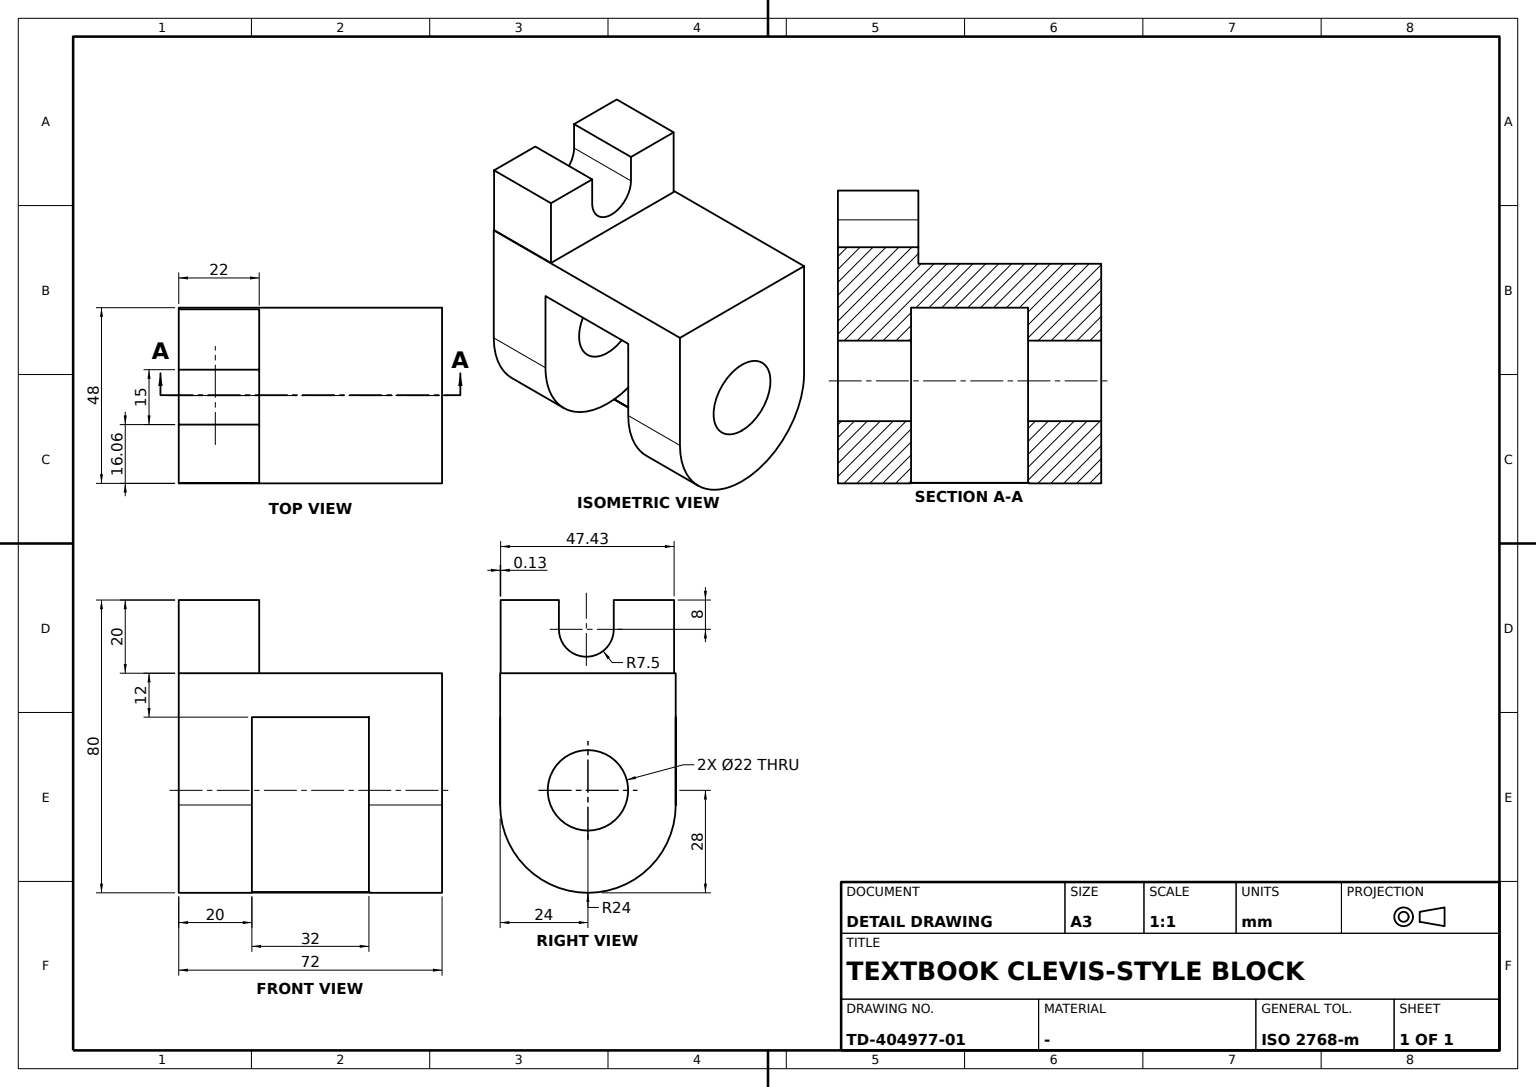
ISO-10303-21;
HEADER;
FILE_DESCRIPTION((''),'2;1');
FILE_NAME('','',(''),(''),'','','');
FILE_SCHEMA(('AUTOMOTIVE_DESIGN'));
ENDSEC;
DATA;
#1=APPLICATION_CONTEXT('');
#2=PRODUCT_CONTEXT('',#1,'mechanical');
#3=PRODUCT('','','',(#2));
#4=PRODUCT_DEFINITION_FORMATION('','',#3);
#5=PRODUCT_DEFINITION_CONTEXT('',#1,'design');
#6=PRODUCT_DEFINITION('','',#4,#5);
#7=PRODUCT_DEFINITION_SHAPE('','',#6);
#8=(LENGTH_UNIT()NAMED_UNIT(*)SI_UNIT(.MILLI.,.METRE.));
#9=(NAMED_UNIT(*)PLANE_ANGLE_UNIT()SI_UNIT($,.RADIAN.));
#10=(NAMED_UNIT(*)SI_UNIT($,.STERADIAN.)SOLID_ANGLE_UNIT());
#11=UNCERTAINTY_MEASURE_WITH_UNIT(LENGTH_MEASURE(0.005),#8,'distance_accuracy_value','');
#12=(GEOMETRIC_REPRESENTATION_CONTEXT(3)GLOBAL_UNCERTAINTY_ASSIGNED_CONTEXT((#11))GLOBAL_UNIT_ASSIGNED_CONTEXT((#8,#9,#10))REPRESENTATION_CONTEXT('',''));
#13=CARTESIAN_POINT('',(16.248648,67.997989,18.815758));
#14=VERTEX_POINT('',#13);
#15=CARTESIAN_POINT('',(16.248648,73.190216,18.813833));
#16=VERTEX_POINT('',#15);
#17=CARTESIAN_POINT('',(16.248648,94.611794,18.815758));
#18=DIRECTION('',(0.,1.,0.));
#19=VECTOR('',#18,1000.);
#20=LINE('',#17,#19);
#21=EDGE_CURVE('',#14,#16,#20,.T.);
#22=ORIENTED_EDGE('',*,*,#21,.T.);
#23=CARTESIAN_POINT('',(16.248648,70.611794,42.673));
#24=DIRECTION('',(-1.,0.,0.));
#25=DIRECTION('',(0.,0.,1.));
#26=AXIS2_PLACEMENT_3D('',#23,#24,#25);
#27=CIRCLE('',#26,24.);
#28=EDGE_CURVE('',#16,#14,#27,.T.);
#29=ORIENTED_EDGE('',*,*,#28,.T.);
#30=EDGE_LOOP('',(#22,#29));
#31=FACE_BOUND('',#30,.T.);
#32=CARTESIAN_POINT('',(16.248648,67.853516,18.815758));
#33=AXIS2_PLACEMENT_3D('',#32,#24,#18);
#34=PLANE('',#33);
#35=ADVANCED_FACE('',(#31),#34,.T.);
#36=CARTESIAN_POINT('',(-16.,70.611794,57.673));
#37=VERTEX_POINT('',#36);
#38=CARTESIAN_POINT('',(-16.,70.611794,46.673));
#39=AXIS2_PLACEMENT_3D('',#38,#24,#25);
#40=CIRCLE('',#39,11.);
#41=EDGE_CURVE('',#37,#37,#40,.T.);
#42=ORIENTED_EDGE('',*,*,#41,.F.);
#43=EDGE_LOOP('',(#42));
#44=FACE_BOUND('',#43,.T.);
#45=CARTESIAN_POINT('',(-36.,70.611794,35.673));
#46=VERTEX_POINT('',#45);
#47=CARTESIAN_POINT('',(-36.,70.611794,46.673));
#48=DIRECTION('',(1.,0.,0.));
#49=DIRECTION('',(0.,0.,-1.));
#50=AXIS2_PLACEMENT_3D('',#47,#48,#49);
#51=CIRCLE('',#50,11.);
#52=EDGE_CURVE('',#46,#46,#51,.T.);
#53=ORIENTED_EDGE('',*,*,#52,.F.);
#54=EDGE_LOOP('',(#53));
#55=FACE_BOUND('',#54,.T.);
#56=CARTESIAN_POINT('',(35.9,70.611794,46.673));
#57=AXIS2_PLACEMENT_3D('',#56,#24,#18);
#58=CYLINDRICAL_SURFACE('',#57,11.);
#59=ADVANCED_FACE('',(#44,#55),#58,.F.);
#60=CARTESIAN_POINT('',(-36.,94.611794,42.673));
#61=VERTEX_POINT('',#60);
#62=CARTESIAN_POINT('',(-36.,94.611794,78.673));
#63=VERTEX_POINT('',#62);
#64=CARTESIAN_POINT('',(-36.,94.611794,0.));
#65=VECTOR('',#25,1000.);
#66=LINE('',#64,#65);
#67=EDGE_CURVE('',#61,#63,#66,.T.);
#68=ORIENTED_EDGE('',*,*,#67,.T.);
#69=CARTESIAN_POINT('',(36.,94.611794,78.673));
#70=VERTEX_POINT('',#69);
#71=CARTESIAN_POINT('',(0.,94.611794,78.673));
#72=VECTOR('',#48,1000.);
#73=LINE('',#71,#72);
#74=EDGE_CURVE('',#63,#70,#73,.T.);
#75=ORIENTED_EDGE('',*,*,#74,.T.);
#76=CARTESIAN_POINT('',(36.,94.611794,42.673));
#77=VERTEX_POINT('',#76);
#78=CARTESIAN_POINT('',(36.,94.611794,0.));
#79=LINE('',#78,#65);
#80=EDGE_CURVE('',#77,#70,#79,.T.);
#81=ORIENTED_EDGE('',*,*,#80,.F.);
#82=CARTESIAN_POINT('',(16.,94.611794,42.673));
#83=VERTEX_POINT('',#82);
#84=CARTESIAN_POINT('',(0.,94.611794,42.673));
#85=LINE('',#84,#72);
#86=EDGE_CURVE('',#83,#77,#85,.T.);
#87=ORIENTED_EDGE('',*,*,#86,.F.);
#88=CARTESIAN_POINT('',(16.,94.611794,66.673));
#89=VERTEX_POINT('',#88);
#90=CARTESIAN_POINT('',(16.,94.611794,18.815758));
#91=LINE('',#90,#65);
#92=EDGE_CURVE('',#83,#89,#91,.T.);
#93=ORIENTED_EDGE('',*,*,#92,.T.);
#94=CARTESIAN_POINT('',(-16.,94.611794,66.673));
#95=VERTEX_POINT('',#94);
#96=VECTOR('',#24,1000.);
#97=LINE('',#88,#96);
#98=EDGE_CURVE('',#89,#95,#97,.T.);
#99=ORIENTED_EDGE('',*,*,#98,.T.);
#100=CARTESIAN_POINT('',(-16.,94.611794,42.673));
#101=VERTEX_POINT('',#100);
#102=VECTOR('',#49,1000.);
#103=LINE('',#94,#102);
#104=EDGE_CURVE('',#95,#101,#103,.T.);
#105=ORIENTED_EDGE('',*,*,#104,.T.);
#106=EDGE_CURVE('',#61,#101,#85,.T.);
#107=ORIENTED_EDGE('',*,*,#106,.F.);
#108=EDGE_LOOP('',(#68,#75,#81,#87,#93,#99,#105,#107));
#109=FACE_BOUND('',#108,.T.);
#110=AXIS2_PLACEMENT_3D('',#84,#18,#25);
#111=PLANE('',#110);
#112=ADVANCED_FACE('',(#109),#111,.T.);
#113=CARTESIAN_POINT('',(-14.,77.672295,90.673));
#114=VERTEX_POINT('',#113);
#115=CARTESIAN_POINT('',(-36.,77.672295,90.673));
#116=VERTEX_POINT('',#115);
#117=CARTESIAN_POINT('',(-25.66,77.672295,90.673));
#118=LINE('',#117,#72);
#119=EDGE_CURVE('',#114,#116,#118,.F.);
#120=ORIENTED_EDGE('',*,*,#119,.T.);
#121=CARTESIAN_POINT('',(-36.,62.672295,90.673));
#122=VERTEX_POINT('',#121);
#123=CARTESIAN_POINT('',(-36.,70.172295,90.673));
#124=AXIS2_PLACEMENT_3D('',#123,#48,#49);
#125=CIRCLE('',#124,7.5);
#126=EDGE_CURVE('',#122,#116,#125,.T.);
#127=ORIENTED_EDGE('',*,*,#126,.F.);
#128=CARTESIAN_POINT('',(-14.,62.672295,90.673));
#129=VERTEX_POINT('',#128);
#130=CARTESIAN_POINT('',(-25.66,62.672295,90.673));
#131=LINE('',#130,#72);
#132=EDGE_CURVE('',#129,#122,#131,.F.);
#133=ORIENTED_EDGE('',*,*,#132,.F.);
#134=CARTESIAN_POINT('',(-14.,70.172295,90.673));
#135=AXIS2_PLACEMENT_3D('',#134,#24,#25);
#136=CIRCLE('',#135,7.5);
#137=EDGE_CURVE('',#129,#114,#136,.F.);
#138=ORIENTED_EDGE('',*,*,#137,.T.);
#139=EDGE_LOOP('',(#120,#127,#133,#138));
#140=FACE_BOUND('',#139,.T.);
#141=CARTESIAN_POINT('',(-25.66,70.172295,90.673));
#142=AXIS2_PLACEMENT_3D('',#141,#48,#18);
#143=CYLINDRICAL_SURFACE('',#142,7.5);
#144=ADVANCED_FACE('',(#140),#143,.F.);
#145=CARTESIAN_POINT('',(36.,70.611794,35.673));
#146=VERTEX_POINT('',#145);
#147=CARTESIAN_POINT('',(36.,70.611794,46.673));
#148=AXIS2_PLACEMENT_3D('',#147,#48,#49);
#149=CIRCLE('',#148,11.);
#150=EDGE_CURVE('',#146,#146,#149,.T.);
#151=ORIENTED_EDGE('',*,*,#150,.T.);
#152=EDGE_LOOP('',(#151));
#153=FACE_BOUND('',#152,.T.);
#154=CARTESIAN_POINT('',(16.,70.611794,35.673));
#155=VERTEX_POINT('',#154);
#156=CARTESIAN_POINT('',(16.,70.611794,46.673));
#157=AXIS2_PLACEMENT_3D('',#156,#48,#49);
#158=CIRCLE('',#157,11.);
#159=EDGE_CURVE('',#155,#155,#158,.T.);
#160=ORIENTED_EDGE('',*,*,#159,.F.);
#161=EDGE_LOOP('',(#160));
#162=FACE_BOUND('',#161,.T.);
#163=ADVANCED_FACE('',(#153,#162),#58,.F.);
#164=ORIENTED_EDGE('',*,*,#159,.T.);
#165=EDGE_LOOP('',(#164));
#166=FACE_BOUND('',#165,.T.);
#167=ORIENTED_EDGE('',*,*,#92,.F.);
#168=CARTESIAN_POINT('',(16.,73.207907,18.815758));
#169=VERTEX_POINT('',#168);
#170=CARTESIAN_POINT('',(16.,70.611794,42.673));
#171=AXIS2_PLACEMENT_3D('',#170,#48,#49);
#172=CIRCLE('',#171,24.);
#173=EDGE_CURVE('',#169,#83,#172,.T.);
#174=ORIENTED_EDGE('',*,*,#173,.F.);
#175=CARTESIAN_POINT('',(16.,67.997989,18.815758));
#176=VERTEX_POINT('',#175);
#177=DIRECTION('',(0.,-1.,0.));
#178=VECTOR('',#177,1000.);
#179=LINE('',#90,#178);
#180=EDGE_CURVE('',#169,#176,#179,.T.);
#181=ORIENTED_EDGE('',*,*,#180,.T.);
#182=CARTESIAN_POINT('',(16.,46.611794,42.673));
#183=VERTEX_POINT('',#182);
#184=EDGE_CURVE('',#183,#176,#172,.T.);
#185=ORIENTED_EDGE('',*,*,#184,.F.);
#186=CARTESIAN_POINT('',(16.,46.611794,66.673));
#187=VERTEX_POINT('',#186);
#188=LINE('',#182,#102);
#189=EDGE_CURVE('',#187,#183,#188,.T.);
#190=ORIENTED_EDGE('',*,*,#189,.F.);
#191=LINE('',#88,#178);
#192=EDGE_CURVE('',#89,#187,#191,.T.);
#193=ORIENTED_EDGE('',*,*,#192,.F.);
#194=EDGE_LOOP('',(#167,#174,#181,#185,#190,#193));
#195=FACE_BOUND('',#194,.T.);
#196=AXIS2_PLACEMENT_3D('',#90,#48,#25);
#197=PLANE('',#196);
#198=ADVANCED_FACE('',(#166,#195),#197,.F.);
#199=ORIENTED_EDGE('',*,*,#192,.T.);
#200=CARTESIAN_POINT('',(-16.,46.611794,66.673));
#201=VERTEX_POINT('',#200);
#202=LINE('',#186,#96);
#203=EDGE_CURVE('',#187,#201,#202,.T.);
#204=ORIENTED_EDGE('',*,*,#203,.T.);
#205=LINE('',#94,#178);
#206=EDGE_CURVE('',#95,#201,#205,.T.);
#207=ORIENTED_EDGE('',*,*,#206,.F.);
#208=ORIENTED_EDGE('',*,*,#98,.F.);
#209=EDGE_LOOP('',(#199,#204,#207,#208));
#210=FACE_BOUND('',#209,.T.);
#211=AXIS2_PLACEMENT_3D('',#88,#25,#24);
#212=PLANE('',#211);
#213=ADVANCED_FACE('',(#210),#212,.F.);
#214=CARTESIAN_POINT('',(-14.,62.672295,98.673));
#215=VERTEX_POINT('',#214);
#216=CARTESIAN_POINT('',(-14.,62.672295,78.673));
#217=LINE('',#216,#65);
#218=EDGE_CURVE('',#129,#215,#217,.T.);
#219=ORIENTED_EDGE('',*,*,#218,.F.);
#220=ORIENTED_EDGE('',*,*,#132,.T.);
#221=CARTESIAN_POINT('',(-36.,62.672295,98.673));
#222=VERTEX_POINT('',#221);
#223=CARTESIAN_POINT('',(-36.,62.672295,0.));
#224=LINE('',#223,#102);
#225=EDGE_CURVE('',#222,#122,#224,.T.);
#226=ORIENTED_EDGE('',*,*,#225,.F.);
#227=LINE('',#214,#96);
#228=EDGE_CURVE('',#215,#222,#227,.T.);
#229=ORIENTED_EDGE('',*,*,#228,.F.);
#230=EDGE_LOOP('',(#219,#220,#226,#229));
#231=FACE_BOUND('',#230,.T.);
#232=AXIS2_PLACEMENT_3D('',#128,#177,#25);
#233=PLANE('',#232);
#234=ADVANCED_FACE('',(#231),#233,.F.);
#235=ORIENTED_EDGE('',*,*,#21,.F.);
#236=LINE('',#175,#72);
#237=EDGE_CURVE('',#176,#14,#236,.T.);
#238=ORIENTED_EDGE('',*,*,#237,.F.);
#239=ORIENTED_EDGE('',*,*,#180,.F.);
#240=CARTESIAN_POINT('',(-16.,73.190216,18.815758));
#241=LINE('',#240,#72);
#242=EDGE_CURVE('',#169,#16,#241,.T.);
#243=ORIENTED_EDGE('',*,*,#242,.T.);
#244=EDGE_LOOP('',(#235,#238,#239,#243));
#245=FACE_BOUND('',#244,.T.);
#246=CARTESIAN_POINT('',(-16.,94.611794,18.815758));
#247=AXIS2_PLACEMENT_3D('',#246,#49,#48);
#248=PLANE('',#247);
#249=ADVANCED_FACE('',(#245),#248,.T.);
#250=CARTESIAN_POINT('',(-16.011372,67.997989,18.815758));
#251=VERTEX_POINT('',#250);
#252=CARTESIAN_POINT('',(-16.,46.611794,42.673));
#253=VERTEX_POINT('',#252);
#254=CARTESIAN_POINT('',(-16.,70.611794,42.673));
#255=AXIS2_PLACEMENT_3D('',#254,#24,#25);
#256=CIRCLE('',#255,24.);
#257=EDGE_CURVE('',#251,#253,#256,.T.);
#258=ORIENTED_EDGE('',*,*,#257,.T.);
#259=CARTESIAN_POINT('',(-36.,46.611794,42.673));
#260=VERTEX_POINT('',#259);
#261=CARTESIAN_POINT('',(0.,46.611794,42.673));
#262=LINE('',#261,#72);
#263=EDGE_CURVE('',#260,#253,#262,.T.);
#264=ORIENTED_EDGE('',*,*,#263,.F.);
#265=CARTESIAN_POINT('',(-36.,70.611794,42.673));
#266=AXIS2_PLACEMENT_3D('',#265,#48,#49);
#267=CIRCLE('',#266,24.);
#268=EDGE_CURVE('',#260,#61,#267,.T.);
#269=ORIENTED_EDGE('',*,*,#268,.T.);
#270=ORIENTED_EDGE('',*,*,#106,.T.);
#271=CARTESIAN_POINT('',(-16.,73.225598,18.815758));
#272=VERTEX_POINT('',#271);
#273=EDGE_CURVE('',#101,#272,#256,.T.);
#274=ORIENTED_EDGE('',*,*,#273,.T.);
#275=LINE('',#271,#72);
#276=EDGE_CURVE('',#272,#169,#275,.T.);
#277=ORIENTED_EDGE('',*,*,#276,.T.);
#278=ORIENTED_EDGE('',*,*,#173,.T.);
#279=ORIENTED_EDGE('',*,*,#86,.T.);
#280=CARTESIAN_POINT('',(36.,46.611794,42.673));
#281=VERTEX_POINT('',#280);
#282=CARTESIAN_POINT('',(36.,70.611794,42.673));
#283=AXIS2_PLACEMENT_3D('',#282,#48,#49);
#284=CIRCLE('',#283,24.);
#285=EDGE_CURVE('',#281,#77,#284,.T.);
#286=ORIENTED_EDGE('',*,*,#285,.F.);
#287=EDGE_CURVE('',#183,#281,#262,.T.);
#288=ORIENTED_EDGE('',*,*,#287,.F.);
#289=ORIENTED_EDGE('',*,*,#184,.T.);
#290=ORIENTED_EDGE('',*,*,#237,.T.);
#291=ORIENTED_EDGE('',*,*,#28,.F.);
#292=CARTESIAN_POINT('',(-16.011372,73.190227,18.813833));
#293=VERTEX_POINT('',#292);
#294=CARTESIAN_POINT('',(-16.011372,73.190216,18.811908));
#295=LINE('',#294,#72);
#296=EDGE_CURVE('',#293,#16,#295,.T.);
#297=ORIENTED_EDGE('',*,*,#296,.F.);
#298=CARTESIAN_POINT('',(-16.022743,70.611794,42.673));
#299=AXIS2_PLACEMENT_3D('',#298,#48,#49);
#300=CIRCLE('',#299,24.);
#301=EDGE_CURVE('',#251,#293,#300,.T.);
#302=ORIENTED_EDGE('',*,*,#301,.F.);
#303=EDGE_LOOP('',(#258,#264,#269,#270,#274,#277,#278,#279,#286,#288,#289,#290,#291,#297,#302));
#304=FACE_BOUND('',#303,.T.);
#305=CARTESIAN_POINT('',(0.,70.611794,42.673));
#306=AXIS2_PLACEMENT_3D('',#305,#48,#18);
#307=CYLINDRICAL_SURFACE('',#306,24.);
#308=ADVANCED_FACE('',(#304),#307,.T.);
#309=ORIENTED_EDGE('',*,*,#119,.F.);
#310=CARTESIAN_POINT('',(-14.,77.672295,98.673));
#311=VERTEX_POINT('',#310);
#312=CARTESIAN_POINT('',(-14.,77.672295,78.673));
#313=LINE('',#312,#65);
#314=EDGE_CURVE('',#114,#311,#313,.T.);
#315=ORIENTED_EDGE('',*,*,#314,.T.);
#316=CARTESIAN_POINT('',(-36.,77.672295,98.673));
#317=VERTEX_POINT('',#316);
#318=LINE('',#310,#96);
#319=EDGE_CURVE('',#311,#317,#318,.T.);
#320=ORIENTED_EDGE('',*,*,#319,.T.);
#321=CARTESIAN_POINT('',(-36.,77.672295,0.));
#322=LINE('',#321,#102);
#323=EDGE_CURVE('',#317,#116,#322,.T.);
#324=ORIENTED_EDGE('',*,*,#323,.T.);
#325=EDGE_LOOP('',(#309,#315,#320,#324));
#326=FACE_BOUND('',#325,.T.);
#327=AXIS2_PLACEMENT_3D('',#113,#177,#25);
#328=PLANE('',#327);
#329=ADVANCED_FACE('',(#326),#328,.T.);
#330=ORIENTED_EDGE('',*,*,#296,.T.);
#331=ORIENTED_EDGE('',*,*,#242,.F.);
#332=EDGE_CURVE('',#293,#169,#241,.T.);
#333=ORIENTED_EDGE('',*,*,#332,.F.);
#334=EDGE_LOOP('',(#330,#331,#333));
#335=FACE_BOUND('',#334,.T.);
#336=CARTESIAN_POINT('',(-16.022743,73.190216,18.815758));
#337=AXIS2_PLACEMENT_3D('',#336,#18,#48);
#338=PLANE('',#337);
#339=ADVANCED_FACE('',(#335),#338,.F.);
#340=CARTESIAN_POINT('',(-14.,94.172295,98.673));
#341=VERTEX_POINT('',#340);
#342=CARTESIAN_POINT('',(-36.,94.172295,98.673));
#343=VERTEX_POINT('',#342);
#344=CARTESIAN_POINT('',(0.,94.172295,98.673));
#345=LINE('',#344,#96);
#346=EDGE_CURVE('',#341,#343,#345,.T.);
#347=ORIENTED_EDGE('',*,*,#346,.T.);
#348=CARTESIAN_POINT('',(-36.,0.,98.673));
#349=LINE('',#348,#19);
#350=EDGE_CURVE('',#317,#343,#349,.T.);
#351=ORIENTED_EDGE('',*,*,#350,.F.);
#352=ORIENTED_EDGE('',*,*,#319,.F.);
#353=CARTESIAN_POINT('',(-14.,0.,98.673));
#354=LINE('',#353,#178);
#355=EDGE_CURVE('',#341,#311,#354,.T.);
#356=ORIENTED_EDGE('',*,*,#355,.F.);
#357=EDGE_LOOP('',(#347,#351,#352,#356));
#358=FACE_BOUND('',#357,.T.);
#359=CARTESIAN_POINT('',(0.,0.,98.673));
#360=AXIS2_PLACEMENT_3D('',#359,#25,#18);
#361=PLANE('',#360);
#362=ADVANCED_FACE('',(#358),#361,.T.);
#363=ORIENTED_EDGE('',*,*,#137,.F.);
#364=ORIENTED_EDGE('',*,*,#218,.T.);
#365=CARTESIAN_POINT('',(-14.,46.738613,98.673));
#366=VERTEX_POINT('',#365);
#367=EDGE_CURVE('',#215,#366,#354,.T.);
#368=ORIENTED_EDGE('',*,*,#367,.T.);
#369=CARTESIAN_POINT('',(-14.,46.738613,78.673));
#370=VERTEX_POINT('',#369);
#371=LINE('',#369,#65);
#372=EDGE_CURVE('',#370,#366,#371,.T.);
#373=ORIENTED_EDGE('',*,*,#372,.F.);
#374=CARTESIAN_POINT('',(-14.,94.172295,78.673));
#375=VERTEX_POINT('',#374);
#376=LINE('',#374,#178);
#377=EDGE_CURVE('',#375,#370,#376,.T.);
#378=ORIENTED_EDGE('',*,*,#377,.F.);
#379=LINE('',#374,#65);
#380=EDGE_CURVE('',#375,#341,#379,.T.);
#381=ORIENTED_EDGE('',*,*,#380,.T.);
#382=ORIENTED_EDGE('',*,*,#355,.T.);
#383=ORIENTED_EDGE('',*,*,#314,.F.);
#384=EDGE_LOOP('',(#363,#364,#368,#373,#378,#381,#382,#383));
#385=FACE_BOUND('',#384,.T.);
#386=AXIS2_PLACEMENT_3D('',#374,#24,#177);
#387=PLANE('',#386);
#388=ADVANCED_FACE('',(#385),#387,.F.);
#389=ORIENTED_EDGE('',*,*,#150,.F.);
#390=EDGE_LOOP('',(#389));
#391=FACE_BOUND('',#390,.T.);
#392=ORIENTED_EDGE('',*,*,#80,.T.);
#393=CARTESIAN_POINT('',(36.,46.611794,78.673));
#394=VERTEX_POINT('',#393);
#395=CARTESIAN_POINT('',(36.,0.,78.673));
#396=LINE('',#395,#19);
#397=EDGE_CURVE('',#394,#70,#396,.T.);
#398=ORIENTED_EDGE('',*,*,#397,.F.);
#399=CARTESIAN_POINT('',(36.,46.611794,0.));
#400=LINE('',#399,#65);
#401=EDGE_CURVE('',#281,#394,#400,.T.);
#402=ORIENTED_EDGE('',*,*,#401,.F.);
#403=ORIENTED_EDGE('',*,*,#285,.T.);
#404=EDGE_LOOP('',(#392,#398,#402,#403));
#405=FACE_BOUND('',#404,.T.);
#406=CARTESIAN_POINT('',(36.,0.,0.));
#407=AXIS2_PLACEMENT_3D('',#406,#48,#18);
#408=PLANE('',#407);
#409=ADVANCED_FACE('',(#391,#405),#408,.T.);
#410=ORIENTED_EDGE('',*,*,#372,.T.);
#411=CARTESIAN_POINT('',(-36.,46.738613,98.673));
#412=VERTEX_POINT('',#411);
#413=CARTESIAN_POINT('',(0.,46.738613,98.673));
#414=LINE('',#413,#72);
#415=EDGE_CURVE('',#412,#366,#414,.T.);
#416=ORIENTED_EDGE('',*,*,#415,.F.);
#417=CARTESIAN_POINT('',(-36.,46.738613,78.673));
#418=VERTEX_POINT('',#417);
#419=LINE('',#417,#65);
#420=EDGE_CURVE('',#418,#412,#419,.T.);
#421=ORIENTED_EDGE('',*,*,#420,.F.);
#422=LINE('',#417,#72);
#423=EDGE_CURVE('',#418,#370,#422,.T.);
#424=ORIENTED_EDGE('',*,*,#423,.T.);
#425=EDGE_LOOP('',(#410,#416,#421,#424));
#426=FACE_BOUND('',#425,.T.);
#427=AXIS2_PLACEMENT_3D('',#417,#177,#48);
#428=PLANE('',#427);
#429=ADVANCED_FACE('',(#426),#428,.T.);
#430=CARTESIAN_POINT('',(-36.,94.172295,78.673));
#431=VERTEX_POINT('',#430);
#432=CARTESIAN_POINT('',(-36.,94.172295,0.));
#433=LINE('',#432,#65);
#434=EDGE_CURVE('',#431,#343,#433,.T.);
#435=ORIENTED_EDGE('',*,*,#434,.T.);
#436=ORIENTED_EDGE('',*,*,#346,.F.);
#437=ORIENTED_EDGE('',*,*,#380,.F.);
#438=LINE('',#374,#96);
#439=EDGE_CURVE('',#375,#431,#438,.T.);
#440=ORIENTED_EDGE('',*,*,#439,.T.);
#441=EDGE_LOOP('',(#435,#436,#437,#440));
#442=FACE_BOUND('',#441,.T.);
#443=AXIS2_PLACEMENT_3D('',#374,#18,#24);
#444=PLANE('',#443);
#445=ADVANCED_FACE('',(#442),#444,.T.);
#446=ORIENTED_EDGE('',*,*,#41,.T.);
#447=EDGE_LOOP('',(#446));
#448=FACE_BOUND('',#447,.T.);
#449=ORIENTED_EDGE('',*,*,#257,.F.);
#450=CARTESIAN_POINT('',(-16.,67.997989,18.815758));
#451=CARTESIAN_POINT('',(-16.,69.728732,18.815758));
#452=CARTESIAN_POINT('',(-16.,71.459474,18.815758));
#453=CARTESIAN_POINT('',(-16.,73.190217,18.815758));
#454=B_SPLINE_CURVE_WITH_KNOTS('',3,(#450,#451,#452,#453),.UNSPECIFIED.,.F.,.F.,(4,4),(21.421577876,26.613806012),.UNSPECIFIED.);
#455=EDGE_CURVE('',#293,#251,#454,.F.);
#456=ORIENTED_EDGE('',*,*,#455,.F.);
#457=LINE('',#246,#178);
#458=EDGE_CURVE('',#272,#293,#457,.T.);
#459=ORIENTED_EDGE('',*,*,#458,.F.);
#460=ORIENTED_EDGE('',*,*,#273,.F.);
#461=ORIENTED_EDGE('',*,*,#104,.F.);
#462=ORIENTED_EDGE('',*,*,#206,.T.);
#463=LINE('',#200,#102);
#464=EDGE_CURVE('',#201,#253,#463,.T.);
#465=ORIENTED_EDGE('',*,*,#464,.T.);
#466=EDGE_LOOP('',(#449,#456,#459,#460,#461,#462,#465));
#467=FACE_BOUND('',#466,.T.);
#468=AXIS2_PLACEMENT_3D('',#94,#24,#49);
#469=PLANE('',#468);
#470=ADVANCED_FACE('',(#448,#467),#469,.F.);
#471=ORIENTED_EDGE('',*,*,#332,.T.);
#472=ORIENTED_EDGE('',*,*,#276,.F.);
#473=ORIENTED_EDGE('',*,*,#458,.T.);
#474=EDGE_LOOP('',(#471,#472,#473));
#475=FACE_BOUND('',#474,.T.);
#476=ADVANCED_FACE('',(#475),#248,.F.);
#477=ORIENTED_EDGE('',*,*,#377,.T.);
#478=ORIENTED_EDGE('',*,*,#423,.F.);
#479=CARTESIAN_POINT('',(-36.,46.611794,78.673));
#480=VERTEX_POINT('',#479);
#481=CARTESIAN_POINT('',(-36.,0.,78.673));
#482=LINE('',#481,#19);
#483=EDGE_CURVE('',#480,#418,#482,.T.);
#484=ORIENTED_EDGE('',*,*,#483,.F.);
#485=CARTESIAN_POINT('',(0.,46.611794,78.673));
#486=LINE('',#485,#72);
#487=EDGE_CURVE('',#480,#394,#486,.T.);
#488=ORIENTED_EDGE('',*,*,#487,.T.);
#489=ORIENTED_EDGE('',*,*,#397,.T.);
#490=ORIENTED_EDGE('',*,*,#74,.F.);
#491=EDGE_CURVE('',#431,#63,#482,.T.);
#492=ORIENTED_EDGE('',*,*,#491,.F.);
#493=ORIENTED_EDGE('',*,*,#439,.F.);
#494=EDGE_LOOP('',(#477,#478,#484,#488,#489,#490,#492,#493));
#495=FACE_BOUND('',#494,.T.);
#496=AXIS2_PLACEMENT_3D('',#485,#49,#18);
#497=PLANE('',#496);
#498=ADVANCED_FACE('',(#495),#497,.F.);
#499=ORIENTED_EDGE('',*,*,#189,.T.);
#500=ORIENTED_EDGE('',*,*,#287,.T.);
#501=ORIENTED_EDGE('',*,*,#401,.T.);
#502=ORIENTED_EDGE('',*,*,#487,.F.);
#503=CARTESIAN_POINT('',(-36.,46.611794,0.));
#504=LINE('',#503,#65);
#505=EDGE_CURVE('',#260,#480,#504,.T.);
#506=ORIENTED_EDGE('',*,*,#505,.F.);
#507=ORIENTED_EDGE('',*,*,#263,.T.);
#508=ORIENTED_EDGE('',*,*,#464,.F.);
#509=ORIENTED_EDGE('',*,*,#203,.F.);
#510=EDGE_LOOP('',(#499,#500,#501,#502,#506,#507,#508,#509));
#511=FACE_BOUND('',#510,.T.);
#512=AXIS2_PLACEMENT_3D('',#261,#18,#25);
#513=PLANE('',#512);
#514=ADVANCED_FACE('',(#511),#513,.F.);
#515=ORIENTED_EDGE('',*,*,#455,.T.);
#516=ORIENTED_EDGE('',*,*,#301,.T.);
#517=EDGE_LOOP('',(#515,#516));
#518=FACE_BOUND('',#517,.T.);
#519=AXIS2_PLACEMENT_3D('',#336,#48,#177);
#520=PLANE('',#519);
#521=ADVANCED_FACE('',(#518),#520,.T.);
#522=ORIENTED_EDGE('',*,*,#52,.T.);
#523=EDGE_LOOP('',(#522));
#524=FACE_BOUND('',#523,.T.);
#525=ORIENTED_EDGE('',*,*,#350,.T.);
#526=ORIENTED_EDGE('',*,*,#434,.F.);
#527=ORIENTED_EDGE('',*,*,#491,.T.);
#528=ORIENTED_EDGE('',*,*,#67,.F.);
#529=ORIENTED_EDGE('',*,*,#268,.F.);
#530=ORIENTED_EDGE('',*,*,#505,.T.);
#531=ORIENTED_EDGE('',*,*,#483,.T.);
#532=ORIENTED_EDGE('',*,*,#420,.T.);
#533=EDGE_CURVE('',#412,#222,#349,.T.);
#534=ORIENTED_EDGE('',*,*,#533,.T.);
#535=ORIENTED_EDGE('',*,*,#225,.T.);
#536=ORIENTED_EDGE('',*,*,#126,.T.);
#537=ORIENTED_EDGE('',*,*,#323,.F.);
#538=EDGE_LOOP('',(#525,#526,#527,#528,#529,#530,#531,#532,#534,#535,#536,#537));
#539=FACE_BOUND('',#538,.T.);
#540=CARTESIAN_POINT('',(-36.,0.,0.));
#541=AXIS2_PLACEMENT_3D('',#540,#48,#18);
#542=PLANE('',#541);
#543=ADVANCED_FACE('',(#524,#539),#542,.F.);
#544=ORIENTED_EDGE('',*,*,#367,.F.);
#545=ORIENTED_EDGE('',*,*,#228,.T.);
#546=ORIENTED_EDGE('',*,*,#533,.F.);
#547=ORIENTED_EDGE('',*,*,#415,.T.);
#548=EDGE_LOOP('',(#544,#545,#546,#547));
#549=FACE_BOUND('',#548,.T.);
#550=ADVANCED_FACE('',(#549),#361,.T.);
#551=CLOSED_SHELL('',(#35,#59,#112,#144,#163,#198,#213,#234,#249,#308,#329,#339,#362,#388,#409,#429,#445,#470,#476,#498,#514,#521,#543,#550));
#552=MANIFOLD_SOLID_BREP('',#551);
#553=ADVANCED_BREP_SHAPE_REPRESENTATION('',(#552),#12);
#554=SHAPE_DEFINITION_REPRESENTATION(#7,#553);
ENDSEC;
END-ISO-10303-21;
